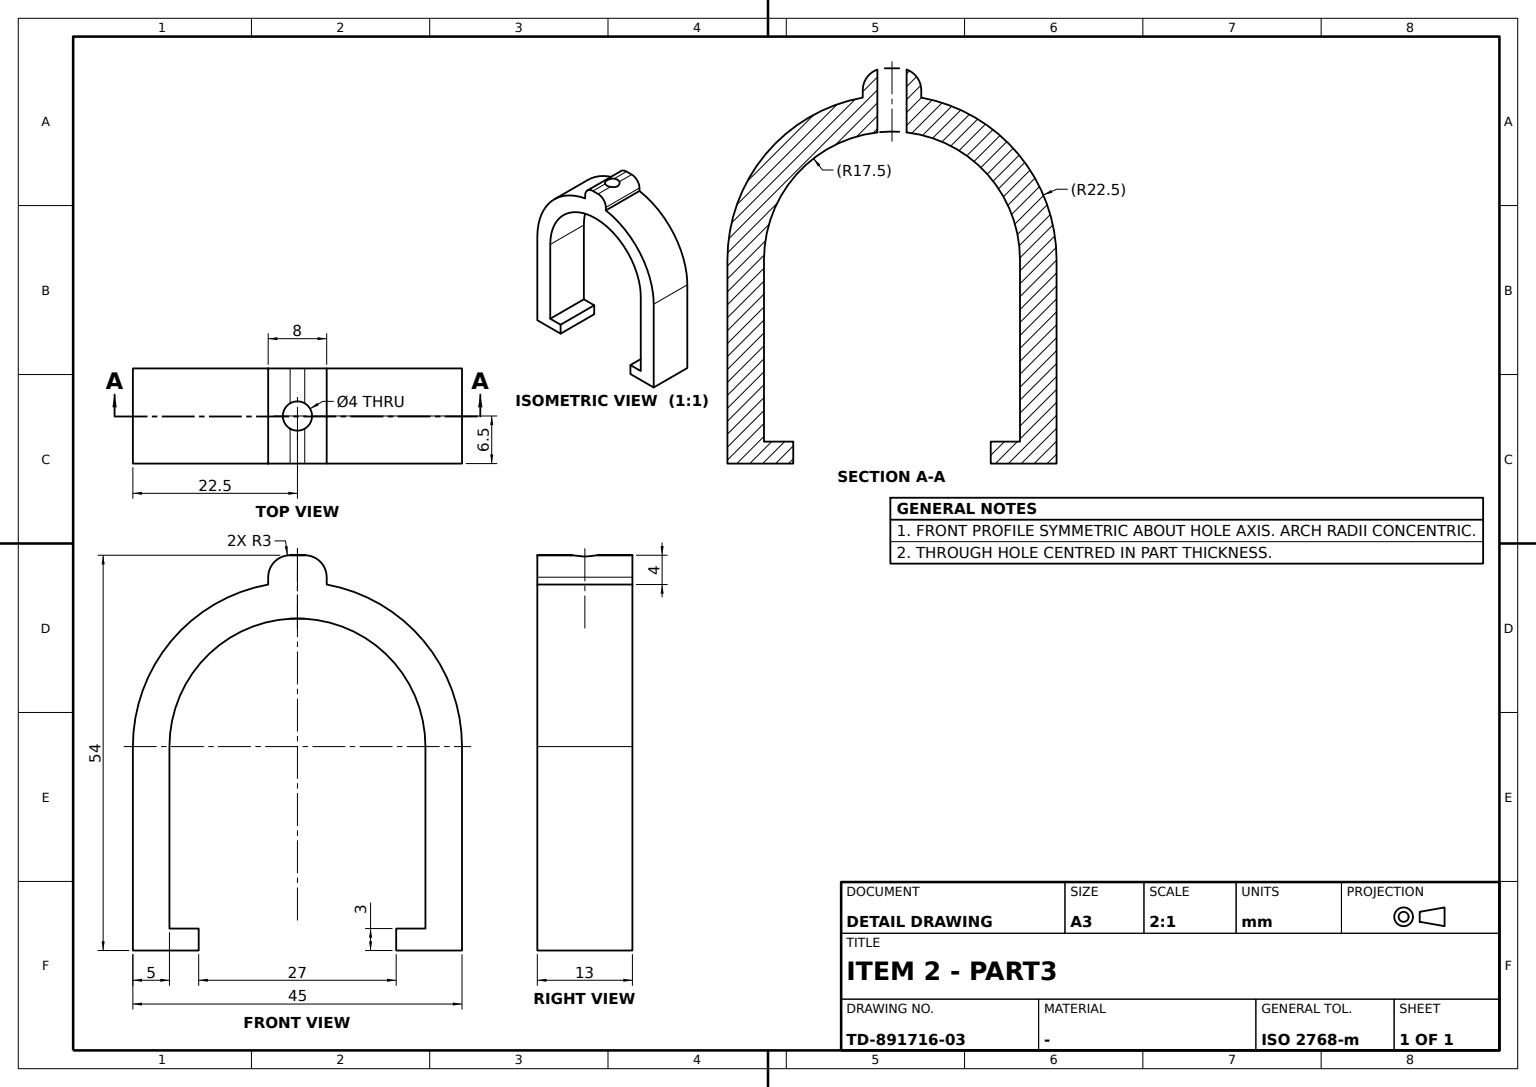
ISO-10303-21;
HEADER;
FILE_DESCRIPTION((''),'2;1');
FILE_NAME('','',(''),(''),'','','');
FILE_SCHEMA(('AUTOMOTIVE_DESIGN'));
ENDSEC;
DATA;
#1=APPLICATION_CONTEXT('');
#2=PRODUCT_CONTEXT('',#1,'mechanical');
#3=PRODUCT('','','',(#2));
#4=PRODUCT_DEFINITION_FORMATION('','',#3);
#5=PRODUCT_DEFINITION_CONTEXT('',#1,'design');
#6=PRODUCT_DEFINITION('','',#4,#5);
#7=PRODUCT_DEFINITION_SHAPE('','',#6);
#8=(LENGTH_UNIT()NAMED_UNIT(*)SI_UNIT(.MILLI.,.METRE.));
#9=(NAMED_UNIT(*)PLANE_ANGLE_UNIT()SI_UNIT($,.RADIAN.));
#10=(NAMED_UNIT(*)SI_UNIT($,.STERADIAN.)SOLID_ANGLE_UNIT());
#11=UNCERTAINTY_MEASURE_WITH_UNIT(LENGTH_MEASURE(0.005),#8,'distance_accuracy_value','');
#12=(GEOMETRIC_REPRESENTATION_CONTEXT(3)GLOBAL_UNCERTAINTY_ASSIGNED_CONTEXT((#11))GLOBAL_UNIT_ASSIGNED_CONTEXT((#8,#9,#10))REPRESENTATION_CONTEXT('',''));
#13=CARTESIAN_POINT('',(4.,0.,50.));
#14=VERTEX_POINT('',#13);
#15=CARTESIAN_POINT('',(4.,0.,51.));
#16=VERTEX_POINT('',#15);
#17=CARTESIAN_POINT('',(4.,0.,0.));
#18=DIRECTION('',(0.,0.,1.));
#19=VECTOR('',#18,1000.);
#20=LINE('',#17,#19);
#21=EDGE_CURVE('',#14,#16,#20,.T.);
#22=ORIENTED_EDGE('',*,*,#21,.F.);
#23=CARTESIAN_POINT('',(4.,13.,50.));
#24=VERTEX_POINT('',#23);
#25=DIRECTION('',(0.,1.,0.));
#26=VECTOR('',#25,1000.);
#27=LINE('',#13,#26);
#28=EDGE_CURVE('',#14,#24,#27,.T.);
#29=ORIENTED_EDGE('',*,*,#28,.T.);
#30=CARTESIAN_POINT('',(4.,13.,51.));
#31=VERTEX_POINT('',#30);
#32=CARTESIAN_POINT('',(4.,13.,0.));
#33=LINE('',#32,#19);
#34=EDGE_CURVE('',#24,#31,#33,.T.);
#35=ORIENTED_EDGE('',*,*,#34,.T.);
#36=CARTESIAN_POINT('',(4.,6.5,51.));
#37=LINE('',#36,#26);
#38=EDGE_CURVE('',#16,#31,#37,.T.);
#39=ORIENTED_EDGE('',*,*,#38,.F.);
#40=EDGE_LOOP('',(#22,#29,#35,#39));
#41=FACE_BOUND('',#40,.T.);
#42=DIRECTION('',(-1.,0.,0.));
#43=AXIS2_PLACEMENT_3D('',#13,#42,#18);
#44=PLANE('',#43);
#45=ADVANCED_FACE('',(#41),#44,.F.);
#46=CARTESIAN_POINT('',(-22.5,13.,27.85841));
#47=VERTEX_POINT('',#46);
#48=CARTESIAN_POINT('',(-4.,13.,50.));
#49=VERTEX_POINT('',#48);
#50=CARTESIAN_POINT('',(0.,13.,27.85841));
#51=AXIS2_PLACEMENT_3D('',#50,#25,#18);
#52=CIRCLE('',#51,22.5);
#53=EDGE_CURVE('',#47,#49,#52,.T.);
#54=ORIENTED_EDGE('',*,*,#53,.F.);
#55=CARTESIAN_POINT('',(-22.5,0.,27.85841));
#56=VERTEX_POINT('',#55);
#57=CARTESIAN_POINT('',(-22.5,6.5,27.85841));
#58=LINE('',#57,#26);
#59=EDGE_CURVE('',#56,#47,#58,.T.);
#60=ORIENTED_EDGE('',*,*,#59,.F.);
#61=CARTESIAN_POINT('',(-4.,0.,50.));
#62=VERTEX_POINT('',#61);
#63=CARTESIAN_POINT('',(0.,0.,27.85841));
#64=AXIS2_PLACEMENT_3D('',#63,#25,#18);
#65=CIRCLE('',#64,22.5);
#66=EDGE_CURVE('',#56,#62,#65,.T.);
#67=ORIENTED_EDGE('',*,*,#66,.T.);
#68=LINE('',#61,#26);
#69=EDGE_CURVE('',#62,#49,#68,.T.);
#70=ORIENTED_EDGE('',*,*,#69,.T.);
#71=EDGE_LOOP('',(#54,#60,#67,#70));
#72=FACE_BOUND('',#71,.T.);
#73=CARTESIAN_POINT('',(0.,6.5,27.85841));
#74=AXIS2_PLACEMENT_3D('',#73,#25,#42);
#75=CYLINDRICAL_SURFACE('',#74,22.5);
#76=ADVANCED_FACE('',(#72),#75,.T.);
#77=CARTESIAN_POINT('',(-4.,13.,51.));
#78=VERTEX_POINT('',#77);
#79=CARTESIAN_POINT('',(-1.,13.,54.));
#80=VERTEX_POINT('',#79);
#81=CARTESIAN_POINT('',(-1.,13.,51.));
#82=AXIS2_PLACEMENT_3D('',#81,#25,#18);
#83=CIRCLE('',#82,3.);
#84=EDGE_CURVE('',#78,#80,#83,.T.);
#85=ORIENTED_EDGE('',*,*,#84,.F.);
#86=CARTESIAN_POINT('',(-4.,0.,51.));
#87=VERTEX_POINT('',#86);
#88=CARTESIAN_POINT('',(-4.,6.5,51.));
#89=LINE('',#88,#26);
#90=EDGE_CURVE('',#87,#78,#89,.T.);
#91=ORIENTED_EDGE('',*,*,#90,.F.);
#92=CARTESIAN_POINT('',(-1.,0.,54.));
#93=VERTEX_POINT('',#92);
#94=CARTESIAN_POINT('',(-1.,0.,51.));
#95=AXIS2_PLACEMENT_3D('',#94,#25,#18);
#96=CIRCLE('',#95,3.);
#97=EDGE_CURVE('',#87,#93,#96,.T.);
#98=ORIENTED_EDGE('',*,*,#97,.T.);
#99=CARTESIAN_POINT('',(-1.,4.767949,54.));
#100=VERTEX_POINT('',#99);
#101=CARTESIAN_POINT('',(-1.,6.5,54.));
#102=LINE('',#101,#26);
#103=EDGE_CURVE('',#93,#100,#102,.T.);
#104=ORIENTED_EDGE('',*,*,#103,.T.);
#105=CARTESIAN_POINT('',(-1.,8.232051,54.));
#106=VERTEX_POINT('',#105);
#107=CARTESIAN_POINT('',(-1.613173,5.121965,54.));
#108=CARTESIAN_POINT('',(-2.386918,6.4984,53.656854));
#109=CARTESIAN_POINT('',(-1.61299,7.878141,54.));
#110=B_SPLINE_CURVE_WITH_KNOTS('',3,(#99,#107,#108,#109,#105),.UNSPECIFIED.,.F.,.F.,(4,1,4),(0.,0.002091024,0.004182047),.UNSPECIFIED.);
#111=EDGE_CURVE('',#100,#106,#110,.T.);
#112=ORIENTED_EDGE('',*,*,#111,.T.);
#113=EDGE_CURVE('',#106,#80,#102,.T.);
#114=ORIENTED_EDGE('',*,*,#113,.T.);
#115=EDGE_LOOP('',(#85,#91,#98,#104,#112,#114));
#116=FACE_BOUND('',#115,.T.);
#117=CARTESIAN_POINT('',(-1.,6.5,51.));
#118=AXIS2_PLACEMENT_3D('',#117,#25,#18);
#119=CYLINDRICAL_SURFACE('',#118,3.);
#120=ADVANCED_FACE('',(#116),#119,.T.);
#121=CARTESIAN_POINT('',(1.,0.,54.));
#122=VERTEX_POINT('',#121);
#123=CARTESIAN_POINT('',(1.,0.,51.));
#124=AXIS2_PLACEMENT_3D('',#123,#25,#18);
#125=CIRCLE('',#124,3.);
#126=EDGE_CURVE('',#122,#16,#125,.T.);
#127=ORIENTED_EDGE('',*,*,#126,.T.);
#128=ORIENTED_EDGE('',*,*,#38,.T.);
#129=CARTESIAN_POINT('',(1.,13.,54.));
#130=VERTEX_POINT('',#129);
#131=CARTESIAN_POINT('',(1.,13.,51.));
#132=AXIS2_PLACEMENT_3D('',#131,#25,#18);
#133=CIRCLE('',#132,3.);
#134=EDGE_CURVE('',#130,#31,#133,.T.);
#135=ORIENTED_EDGE('',*,*,#134,.F.);
#136=CARTESIAN_POINT('',(1.,8.232051,54.));
#137=VERTEX_POINT('',#136);
#138=CARTESIAN_POINT('',(1.,6.5,54.));
#139=LINE('',#138,#26);
#140=EDGE_CURVE('',#137,#130,#139,.T.);
#141=ORIENTED_EDGE('',*,*,#140,.F.);
#142=CARTESIAN_POINT('',(1.,4.767949,54.));
#143=VERTEX_POINT('',#142);
#144=CARTESIAN_POINT('',(1.613173,5.121965,54.));
#145=CARTESIAN_POINT('',(2.386918,6.4984,53.656854));
#146=CARTESIAN_POINT('',(1.61299,7.878141,54.));
#147=B_SPLINE_CURVE_WITH_KNOTS('',3,(#142,#144,#145,#146,#136),.UNSPECIFIED.,.F.,.F.,(4,1,4),(0.,0.002091024,0.004182047),.UNSPECIFIED.);
#148=EDGE_CURVE('',#143,#137,#147,.T.);
#149=ORIENTED_EDGE('',*,*,#148,.F.);
#150=EDGE_CURVE('',#122,#143,#139,.T.);
#151=ORIENTED_EDGE('',*,*,#150,.F.);
#152=EDGE_LOOP('',(#127,#128,#135,#141,#149,#151));
#153=FACE_BOUND('',#152,.T.);
#154=CARTESIAN_POINT('',(1.,6.5,51.));
#155=DIRECTION('',(1.,0.,0.));
#156=AXIS2_PLACEMENT_3D('',#154,#25,#155);
#157=CYLINDRICAL_SURFACE('',#156,3.);
#158=ADVANCED_FACE('',(#153),#157,.T.);
#159=CARTESIAN_POINT('',(22.5,0.,0.));
#160=VERTEX_POINT('',#159);
#161=CARTESIAN_POINT('',(22.5,13.,0.));
#162=VERTEX_POINT('',#161);
#163=LINE('',#159,#26);
#164=EDGE_CURVE('',#160,#162,#163,.T.);
#165=ORIENTED_EDGE('',*,*,#164,.F.);
#166=CARTESIAN_POINT('',(13.5,0.,0.));
#167=VERTEX_POINT('',#166);
#168=CARTESIAN_POINT('',(0.,0.,0.));
#169=VECTOR('',#155,1000.);
#170=LINE('',#168,#169);
#171=EDGE_CURVE('',#167,#160,#170,.T.);
#172=ORIENTED_EDGE('',*,*,#171,.F.);
#173=CARTESIAN_POINT('',(13.5,13.,0.));
#174=VERTEX_POINT('',#173);
#175=LINE('',#166,#26);
#176=EDGE_CURVE('',#167,#174,#175,.T.);
#177=ORIENTED_EDGE('',*,*,#176,.T.);
#178=CARTESIAN_POINT('',(0.,13.,0.));
#179=LINE('',#178,#169);
#180=EDGE_CURVE('',#174,#162,#179,.T.);
#181=ORIENTED_EDGE('',*,*,#180,.T.);
#182=EDGE_LOOP('',(#165,#172,#177,#181));
#183=FACE_BOUND('',#182,.T.);
#184=CARTESIAN_POINT('',(-22.5,0.,0.));
#185=AXIS2_PLACEMENT_3D('',#184,#18,#155);
#186=PLANE('',#185);
#187=ADVANCED_FACE('',(#183),#186,.F.);
#188=CARTESIAN_POINT('',(17.5,0.,3.));
#189=VERTEX_POINT('',#188);
#190=CARTESIAN_POINT('',(17.5,13.,3.));
#191=VERTEX_POINT('',#190);
#192=LINE('',#188,#26);
#193=EDGE_CURVE('',#189,#191,#192,.T.);
#194=ORIENTED_EDGE('',*,*,#193,.F.);
#195=CARTESIAN_POINT('',(17.5,0.,27.85841));
#196=VERTEX_POINT('',#195);
#197=CARTESIAN_POINT('',(17.5,0.,0.));
#198=DIRECTION('',(0.,0.,-1.));
#199=VECTOR('',#198,1000.);
#200=LINE('',#197,#199);
#201=EDGE_CURVE('',#196,#189,#200,.T.);
#202=ORIENTED_EDGE('',*,*,#201,.F.);
#203=CARTESIAN_POINT('',(17.5,13.,27.85841));
#204=VERTEX_POINT('',#203);
#205=CARTESIAN_POINT('',(17.5,6.5,27.85841));
#206=LINE('',#205,#26);
#207=EDGE_CURVE('',#196,#204,#206,.T.);
#208=ORIENTED_EDGE('',*,*,#207,.T.);
#209=CARTESIAN_POINT('',(17.5,13.,0.));
#210=LINE('',#209,#199);
#211=EDGE_CURVE('',#204,#191,#210,.T.);
#212=ORIENTED_EDGE('',*,*,#211,.T.);
#213=EDGE_LOOP('',(#194,#202,#208,#212));
#214=FACE_BOUND('',#213,.T.);
#215=AXIS2_PLACEMENT_3D('',#195,#155,#198);
#216=PLANE('',#215);
#217=ADVANCED_FACE('',(#214),#216,.F.);
#218=ORIENTED_EDGE('',*,*,#69,.F.);
#219=CARTESIAN_POINT('',(-4.,0.,0.));
#220=LINE('',#219,#199);
#221=EDGE_CURVE('',#87,#62,#220,.T.);
#222=ORIENTED_EDGE('',*,*,#221,.F.);
#223=ORIENTED_EDGE('',*,*,#90,.T.);
#224=CARTESIAN_POINT('',(-4.,13.,0.));
#225=LINE('',#224,#199);
#226=EDGE_CURVE('',#78,#49,#225,.T.);
#227=ORIENTED_EDGE('',*,*,#226,.T.);
#228=EDGE_LOOP('',(#218,#222,#223,#227));
#229=FACE_BOUND('',#228,.T.);
#230=CARTESIAN_POINT('',(-4.,0.,54.));
#231=AXIS2_PLACEMENT_3D('',#230,#155,#198);
#232=PLANE('',#231);
#233=ADVANCED_FACE('',(#229),#232,.F.);
#234=CARTESIAN_POINT('',(-17.5,0.,3.));
#235=VERTEX_POINT('',#234);
#236=CARTESIAN_POINT('',(-17.5,13.,3.));
#237=VERTEX_POINT('',#236);
#238=LINE('',#234,#26);
#239=EDGE_CURVE('',#235,#237,#238,.T.);
#240=ORIENTED_EDGE('',*,*,#239,.F.);
#241=CARTESIAN_POINT('',(-13.5,0.,3.));
#242=VERTEX_POINT('',#241);
#243=CARTESIAN_POINT('',(0.,0.,3.));
#244=VECTOR('',#42,1000.);
#245=LINE('',#243,#244);
#246=EDGE_CURVE('',#242,#235,#245,.T.);
#247=ORIENTED_EDGE('',*,*,#246,.F.);
#248=CARTESIAN_POINT('',(-13.5,13.,3.));
#249=VERTEX_POINT('',#248);
#250=LINE('',#241,#26);
#251=EDGE_CURVE('',#242,#249,#250,.T.);
#252=ORIENTED_EDGE('',*,*,#251,.T.);
#253=CARTESIAN_POINT('',(0.,13.,3.));
#254=LINE('',#253,#244);
#255=EDGE_CURVE('',#249,#237,#254,.T.);
#256=ORIENTED_EDGE('',*,*,#255,.T.);
#257=EDGE_LOOP('',(#240,#247,#252,#256));
#258=FACE_BOUND('',#257,.T.);
#259=AXIS2_PLACEMENT_3D('',#188,#198,#42);
#260=PLANE('',#259);
#261=ADVANCED_FACE('',(#258),#260,.F.);
#262=ORIENTED_EDGE('',*,*,#164,.T.);
#263=CARTESIAN_POINT('',(22.5,13.,27.85841));
#264=VERTEX_POINT('',#263);
#265=LINE('',#161,#19);
#266=EDGE_CURVE('',#162,#264,#265,.T.);
#267=ORIENTED_EDGE('',*,*,#266,.T.);
#268=CARTESIAN_POINT('',(22.5,0.,27.85841));
#269=VERTEX_POINT('',#268);
#270=CARTESIAN_POINT('',(22.5,6.5,27.85841));
#271=LINE('',#270,#26);
#272=EDGE_CURVE('',#269,#264,#271,.T.);
#273=ORIENTED_EDGE('',*,*,#272,.F.);
#274=LINE('',#159,#19);
#275=EDGE_CURVE('',#160,#269,#274,.T.);
#276=ORIENTED_EDGE('',*,*,#275,.F.);
#277=EDGE_LOOP('',(#262,#267,#273,#276));
#278=FACE_BOUND('',#277,.T.);
#279=AXIS2_PLACEMENT_3D('',#159,#42,#18);
#280=PLANE('',#279);
#281=ADVANCED_FACE('',(#278),#280,.F.);
#282=CARTESIAN_POINT('',(0.,4.5,45.35841));
#283=VERTEX_POINT('',#282);
#284=CARTESIAN_POINT('',(-1.568833,4.933771,45.301134));
#285=CARTESIAN_POINT('',(0.000388,4.283195,45.387021));
#286=CARTESIAN_POINT('',(1.56728,4.933449,45.301244));
#287=CARTESIAN_POINT('',(2.215971,6.497924,45.215029));
#288=CARTESIAN_POINT('',(1.568832,8.066232,45.301134));
#289=CARTESIAN_POINT('',(-0.000396,8.716805,45.387021));
#290=CARTESIAN_POINT('',(-1.567281,8.066548,45.301244));
#291=CARTESIAN_POINT('',(-2.215971,6.502076,45.215029));
#292=B_SPLINE_CURVE_WITH_KNOTS('',3,(#284,#285,#286,#287,#288,#289,#290,#291,#284,#285,#286),.UNSPECIFIED.,.T.,.F.,(1,1,1,1,1,1,1,1,1,1,1,1,1,1,1),(-0.004692459,-0.003128306,-0.001564153,0.,0.001564153,0.003128306,0.004692459,0.006256613,0.007820766,0.009384919,0.010949072,0.012513225,0.014077378,0.015641531,0.017205684),.UNSPECIFIED.);
#293=EDGE_CURVE('',#283,#283,#292,.T.);
#294=ORIENTED_EDGE('',*,*,#293,.F.);
#295=EDGE_LOOP('',(#294));
#296=FACE_BOUND('',#295,.T.);
#297=ORIENTED_EDGE('',*,*,#111,.F.);
#298=CARTESIAN_POINT('',(0.,6.5,54.));
#299=AXIS2_PLACEMENT_3D('',#298,#198,#42);
#300=CIRCLE('',#299,2.);
#301=EDGE_CURVE('',#100,#143,#300,.F.);
#302=ORIENTED_EDGE('',*,*,#301,.T.);
#303=ORIENTED_EDGE('',*,*,#148,.T.);
#304=EDGE_CURVE('',#137,#106,#300,.F.);
#305=ORIENTED_EDGE('',*,*,#304,.T.);
#306=EDGE_LOOP('',(#297,#302,#303,#305));
#307=FACE_BOUND('',#306,.T.);
#308=CARTESIAN_POINT('',(0.,6.5,47.5));
#309=AXIS2_PLACEMENT_3D('',#308,#18,#25);
#310=CYLINDRICAL_SURFACE('',#309,2.);
#311=ADVANCED_FACE('',(#296,#307),#310,.F.);
#312=ORIENTED_EDGE('',*,*,#193,.T.);
#313=CARTESIAN_POINT('',(13.5,13.,3.));
#314=VERTEX_POINT('',#313);
#315=EDGE_CURVE('',#191,#314,#254,.T.);
#316=ORIENTED_EDGE('',*,*,#315,.T.);
#317=CARTESIAN_POINT('',(13.5,0.,3.));
#318=VERTEX_POINT('',#317);
#319=LINE('',#317,#26);
#320=EDGE_CURVE('',#318,#314,#319,.T.);
#321=ORIENTED_EDGE('',*,*,#320,.F.);
#322=EDGE_CURVE('',#189,#318,#245,.T.);
#323=ORIENTED_EDGE('',*,*,#322,.F.);
#324=EDGE_LOOP('',(#312,#316,#321,#323));
#325=FACE_BOUND('',#324,.T.);
#326=ADVANCED_FACE('',(#325),#260,.F.);
#327=ORIENTED_EDGE('',*,*,#150,.T.);
#328=ORIENTED_EDGE('',*,*,#301,.F.);
#329=ORIENTED_EDGE('',*,*,#103,.F.);
#330=CARTESIAN_POINT('',(0.,0.,54.));
#331=LINE('',#330,#244);
#332=EDGE_CURVE('',#122,#93,#331,.T.);
#333=ORIENTED_EDGE('',*,*,#332,.F.);
#334=EDGE_LOOP('',(#327,#328,#329,#333));
#335=FACE_BOUND('',#334,.T.);
#336=CARTESIAN_POINT('',(4.,0.,54.));
#337=AXIS2_PLACEMENT_3D('',#336,#198,#42);
#338=PLANE('',#337);
#339=ADVANCED_FACE('',(#335),#338,.F.);
#340=CARTESIAN_POINT('',(-17.5,0.,27.85841));
#341=VERTEX_POINT('',#340);
#342=CARTESIAN_POINT('',(-17.5,13.,27.85841));
#343=VERTEX_POINT('',#342);
#344=CARTESIAN_POINT('',(-17.5,6.5,27.85841));
#345=LINE('',#344,#26);
#346=EDGE_CURVE('',#341,#343,#345,.T.);
#347=ORIENTED_EDGE('',*,*,#346,.T.);
#348=CIRCLE('',#51,17.5);
#349=EDGE_CURVE('',#343,#204,#348,.T.);
#350=ORIENTED_EDGE('',*,*,#349,.T.);
#351=ORIENTED_EDGE('',*,*,#207,.F.);
#352=CIRCLE('',#64,17.5);
#353=EDGE_CURVE('',#341,#196,#352,.T.);
#354=ORIENTED_EDGE('',*,*,#353,.F.);
#355=EDGE_LOOP('',(#347,#350,#351,#354));
#356=FACE_BOUND('',#355,.T.);
#357=ORIENTED_EDGE('',*,*,#293,.T.);
#358=EDGE_LOOP('',(#357));
#359=FACE_BOUND('',#358,.T.);
#360=CYLINDRICAL_SURFACE('',#74,17.5);
#361=ADVANCED_FACE('',(#356,#359),#360,.F.);
#362=CARTESIAN_POINT('',(-13.5,13.,0.));
#363=VERTEX_POINT('',#362);
#364=LINE('',#362,#19);
#365=EDGE_CURVE('',#363,#249,#364,.T.);
#366=ORIENTED_EDGE('',*,*,#365,.T.);
#367=ORIENTED_EDGE('',*,*,#251,.F.);
#368=CARTESIAN_POINT('',(-13.5,0.,0.));
#369=VERTEX_POINT('',#368);
#370=LINE('',#368,#19);
#371=EDGE_CURVE('',#369,#242,#370,.T.);
#372=ORIENTED_EDGE('',*,*,#371,.F.);
#373=LINE('',#368,#26);
#374=EDGE_CURVE('',#369,#363,#373,.T.);
#375=ORIENTED_EDGE('',*,*,#374,.T.);
#376=EDGE_LOOP('',(#366,#367,#372,#375));
#377=FACE_BOUND('',#376,.T.);
#378=AXIS2_PLACEMENT_3D('',#368,#42,#18);
#379=PLANE('',#378);
#380=ADVANCED_FACE('',(#377),#379,.F.);
#381=ORIENTED_EDGE('',*,*,#84,.T.);
#382=CARTESIAN_POINT('',(0.,13.,54.));
#383=LINE('',#382,#244);
#384=EDGE_CURVE('',#130,#80,#383,.T.);
#385=ORIENTED_EDGE('',*,*,#384,.F.);
#386=ORIENTED_EDGE('',*,*,#134,.T.);
#387=ORIENTED_EDGE('',*,*,#34,.F.);
#388=EDGE_CURVE('',#24,#264,#52,.T.);
#389=ORIENTED_EDGE('',*,*,#388,.T.);
#390=ORIENTED_EDGE('',*,*,#266,.F.);
#391=ORIENTED_EDGE('',*,*,#180,.F.);
#392=LINE('',#173,#199);
#393=EDGE_CURVE('',#314,#174,#392,.T.);
#394=ORIENTED_EDGE('',*,*,#393,.F.);
#395=ORIENTED_EDGE('',*,*,#315,.F.);
#396=ORIENTED_EDGE('',*,*,#211,.F.);
#397=ORIENTED_EDGE('',*,*,#349,.F.);
#398=CARTESIAN_POINT('',(-17.5,13.,0.));
#399=LINE('',#398,#19);
#400=EDGE_CURVE('',#237,#343,#399,.T.);
#401=ORIENTED_EDGE('',*,*,#400,.F.);
#402=ORIENTED_EDGE('',*,*,#255,.F.);
#403=ORIENTED_EDGE('',*,*,#365,.F.);
#404=CARTESIAN_POINT('',(-22.5,13.,0.));
#405=VERTEX_POINT('',#404);
#406=EDGE_CURVE('',#405,#363,#179,.T.);
#407=ORIENTED_EDGE('',*,*,#406,.F.);
#408=LINE('',#404,#199);
#409=EDGE_CURVE('',#47,#405,#408,.T.);
#410=ORIENTED_EDGE('',*,*,#409,.F.);
#411=ORIENTED_EDGE('',*,*,#53,.T.);
#412=ORIENTED_EDGE('',*,*,#226,.F.);
#413=EDGE_LOOP('',(#381,#385,#386,#387,#389,#390,#391,#394,#395,#396,#397,#401,#402,#403,#407,#410,#411,#412));
#414=FACE_BOUND('',#413,.T.);
#415=AXIS2_PLACEMENT_3D('',#178,#25,#42);
#416=PLANE('',#415);
#417=ADVANCED_FACE('',(#414),#416,.T.);
#418=ORIENTED_EDGE('',*,*,#320,.T.);
#419=ORIENTED_EDGE('',*,*,#393,.T.);
#420=ORIENTED_EDGE('',*,*,#176,.F.);
#421=LINE('',#166,#199);
#422=EDGE_CURVE('',#318,#167,#421,.T.);
#423=ORIENTED_EDGE('',*,*,#422,.F.);
#424=EDGE_LOOP('',(#418,#419,#420,#423));
#425=FACE_BOUND('',#424,.T.);
#426=AXIS2_PLACEMENT_3D('',#317,#155,#198);
#427=PLANE('',#426);
#428=ADVANCED_FACE('',(#425),#427,.F.);
#429=ORIENTED_EDGE('',*,*,#332,.T.);
#430=ORIENTED_EDGE('',*,*,#97,.F.);
#431=ORIENTED_EDGE('',*,*,#221,.T.);
#432=ORIENTED_EDGE('',*,*,#66,.F.);
#433=VERTEX_POINT('',#184);
#434=LINE('',#184,#199);
#435=EDGE_CURVE('',#56,#433,#434,.T.);
#436=ORIENTED_EDGE('',*,*,#435,.T.);
#437=EDGE_CURVE('',#433,#369,#170,.T.);
#438=ORIENTED_EDGE('',*,*,#437,.T.);
#439=ORIENTED_EDGE('',*,*,#371,.T.);
#440=ORIENTED_EDGE('',*,*,#246,.T.);
#441=CARTESIAN_POINT('',(-17.5,0.,0.));
#442=LINE('',#441,#19);
#443=EDGE_CURVE('',#235,#341,#442,.T.);
#444=ORIENTED_EDGE('',*,*,#443,.T.);
#445=ORIENTED_EDGE('',*,*,#353,.T.);
#446=ORIENTED_EDGE('',*,*,#201,.T.);
#447=ORIENTED_EDGE('',*,*,#322,.T.);
#448=ORIENTED_EDGE('',*,*,#422,.T.);
#449=ORIENTED_EDGE('',*,*,#171,.T.);
#450=ORIENTED_EDGE('',*,*,#275,.T.);
#451=EDGE_CURVE('',#14,#269,#65,.T.);
#452=ORIENTED_EDGE('',*,*,#451,.F.);
#453=ORIENTED_EDGE('',*,*,#21,.T.);
#454=ORIENTED_EDGE('',*,*,#126,.F.);
#455=EDGE_LOOP('',(#429,#430,#431,#432,#436,#438,#439,#440,#444,#445,#446,#447,#448,#449,#450,#452,#453,#454));
#456=FACE_BOUND('',#455,.T.);
#457=AXIS2_PLACEMENT_3D('',#168,#25,#42);
#458=PLANE('',#457);
#459=ADVANCED_FACE('',(#456),#458,.F.);
#460=ORIENTED_EDGE('',*,*,#113,.F.);
#461=ORIENTED_EDGE('',*,*,#304,.F.);
#462=ORIENTED_EDGE('',*,*,#140,.T.);
#463=ORIENTED_EDGE('',*,*,#384,.T.);
#464=EDGE_LOOP('',(#460,#461,#462,#463));
#465=FACE_BOUND('',#464,.T.);
#466=ADVANCED_FACE('',(#465),#338,.F.);
#467=ORIENTED_EDGE('',*,*,#374,.F.);
#468=ORIENTED_EDGE('',*,*,#437,.F.);
#469=LINE('',#184,#26);
#470=EDGE_CURVE('',#433,#405,#469,.T.);
#471=ORIENTED_EDGE('',*,*,#470,.T.);
#472=ORIENTED_EDGE('',*,*,#406,.T.);
#473=EDGE_LOOP('',(#467,#468,#471,#472));
#474=FACE_BOUND('',#473,.T.);
#475=ADVANCED_FACE('',(#474),#186,.F.);
#476=ORIENTED_EDGE('',*,*,#443,.F.);
#477=ORIENTED_EDGE('',*,*,#239,.T.);
#478=ORIENTED_EDGE('',*,*,#400,.T.);
#479=ORIENTED_EDGE('',*,*,#346,.F.);
#480=EDGE_LOOP('',(#476,#477,#478,#479));
#481=FACE_BOUND('',#480,.T.);
#482=AXIS2_PLACEMENT_3D('',#234,#42,#18);
#483=PLANE('',#482);
#484=ADVANCED_FACE('',(#481),#483,.F.);
#485=ORIENTED_EDGE('',*,*,#435,.F.);
#486=ORIENTED_EDGE('',*,*,#59,.T.);
#487=ORIENTED_EDGE('',*,*,#409,.T.);
#488=ORIENTED_EDGE('',*,*,#470,.F.);
#489=EDGE_LOOP('',(#485,#486,#487,#488));
#490=FACE_BOUND('',#489,.T.);
#491=AXIS2_PLACEMENT_3D('',#55,#155,#198);
#492=PLANE('',#491);
#493=ADVANCED_FACE('',(#490),#492,.F.);
#494=ORIENTED_EDGE('',*,*,#451,.T.);
#495=ORIENTED_EDGE('',*,*,#272,.T.);
#496=ORIENTED_EDGE('',*,*,#388,.F.);
#497=ORIENTED_EDGE('',*,*,#28,.F.);
#498=EDGE_LOOP('',(#494,#495,#496,#497));
#499=FACE_BOUND('',#498,.T.);
#500=ADVANCED_FACE('',(#499),#75,.T.);
#501=CLOSED_SHELL('',(#45,#76,#120,#158,#187,#217,#233,#261,#281,#311,#326,#339,#361,#380,#417,#428,#459,#466,#475,#484,#493,#500));
#502=MANIFOLD_SOLID_BREP('',#501);
#503=ADVANCED_BREP_SHAPE_REPRESENTATION('',(#502),#12);
#504=SHAPE_DEFINITION_REPRESENTATION(#7,#503);
ENDSEC;
END-ISO-10303-21;
